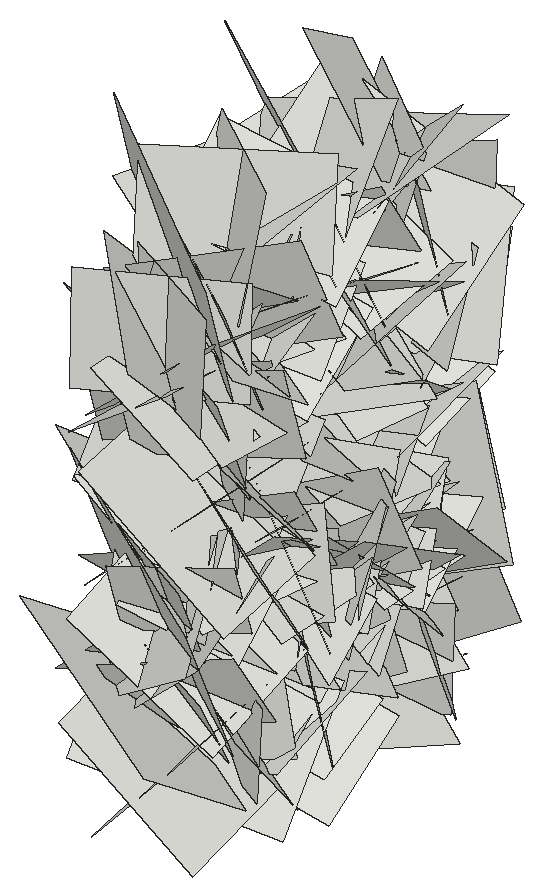
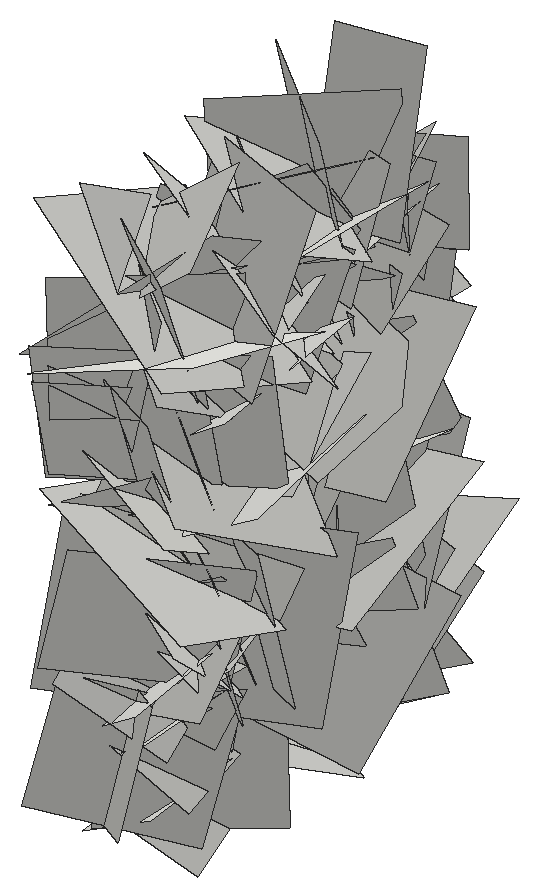
# SketchUp Ruby script. Lengths in inches.
U = 1.inch
M = Sketchup.active_model
def pt(a) = Geom::Point3d.new(a.map { |v| v * U })
def face(e, loops, mat)
  f = e.add_face(loops[0].map { |a| pt(a) })
  loops[1..].each { |l| e.add_face(l.map { |a| pt(a) }).erase! }
  f.material = f.back_material = mat if mat
  f
end
# faces: each face lists its corners as indices into pts; further lists are holes
def faces(e, pts, list, mat = nil) = list.each { |f| face(e, (f[0].is_a?(Array) ? f : [f]).map { |l| l.map { |i| pts[i] } }, mat) }
# xy, xz, yz: faces in a plane at the given z, y or x. An outline is a flat list of corners, or four numbers for a rectangle; further outlines are holes
def ring(l) = l.size == 4 ? [[l[0], l[1]], [l[2], l[1]], [l[2], l[3]], [l[0], l[3]]] : l.each_slice(2).to_a
def flat(e, list, mat, &to3) = list.each { |f| face(e, (f[0].is_a?(Array) ? f : [f]).map { |l| ring(l).map { |u, v| to3.(u, v) } }, mat) }
def xy(e, z, list, mat = nil) = flat(e, list, mat) { |x, y| [x, y, z] }
def xz(e, y, list, mat = nil) = flat(e, list, mat) { |x, z| [x, y, z] }
def yz(e, x, list, mat = nil) = flat(e, list, mat) { |y, z| [x, y, z] }
def lines(e, pts, list) = list.each { |a, b| e.add_line(pt(pts[a]), pt(pts[b])) }
# prism: a flat outline (further loops are holes) pulled along v
def prism(e, loops, v, mat = nil)
  f = face(e, loops, mat); d = Geom::Vector3d.new(v.map { |x| x * U })
  f.pushpull(f.normal.samedirection?(d) ? d.length : -d.length)
end
def box(e, o, s, mat = nil) = prism(e, [[o, [o[0] + s[0], o[1], o[2]], [o[0] + s[0], o[1] + s[1], o[2]], [o[0], o[1] + s[1], o[2]]]], [0, 0, s[2]], mat)
def at(x, y, z, deg = 0) = Geom::Transformation.translation(pt([x, y, z])) * Geom::Transformation.rotation(ORIGIN, Z_AXIS, deg.degrees)
def axes(o, x, y, z) = Geom::Transformation.new([*x, 0, *y, 0, *z, 0, *pt(o).to_a, 1])
def part(name) = M.definitions.add(name)
# library, detail: a bought-in or finely detailed component or shape, given as its bounding box
def library(name, o, s) = part(name).tap { |d| box(d.entities, o, s) }
def detail(e, o, s) = box(e.add_group.entities, o, s)
def put(e, d, t, mat = nil) = e.add_instance(d, t).tap { |i| i.material = mat if mat }
def group(e, t, mat = nil) = e.add_group.tap { |g| g.transformation = t; g.material = mat if mat }.entities
root = M.entities
c1 = part("Component\#6")
p = [[0.01,0,0],[0,3.24,4.54],[4.32,3.24,4.54],[4.33,0,0]]
faces(c1.entities,p,[[0,1,2,3]])
put(root,c1,axes([18.5,153.14,23.91],[-0.18,-1.08552,0.79109],[-0.08355,0.80406,1.08641],[-1.42134,0.0902,-0.16405]))
put(root,c1,axes([18.5,153.125,28.17],[0.03085,-0.9293,0.97672],[-0.26234,0.95667,0.91759],[-1.40479,-0.19906,-0.14991]))
put(root,c1,axes([18.5,153.73,28.3],[0.01858,0.99462,-0.84655],[-0.29457,-0.8244,-0.97435],[-1.35277,0.19318,0.20054]))
put(root,c1,axes([18.5,161.74,34.71],[-0.1652,-1.10091,-0.16395],[-0.26327,-0.12698,1.08875],[-1.15009,0.1872,-0.22568]))
put(root,c1,axes([18.5,157.5625,26.25],[-0.15158,-0.38022,-1.22414],[0.0526,-1.23246,0.37701],[-1.35773,-0.0053,0.15127]))
put(root,c1,axes([18.5,156.14,33.68],[-0.06217,-0.55405,1.15944],[-0.03014,1.16092,0.55332],[-1.36179,-0.0004,-0.06518]))
put(root,c1,axes([18.5,153.92,36.42],[-0.14295,0.82362,0.79821],[-0.11339,0.79118,-0.83443],[-1.21047,-0.17138,-0.0161]))
put(root,c1,axes([18.5,149.67,23.37],[0.09539,-0.59855,1.14231],[-0.08783,1.14003,0.60389],[-1.36418,-0.11525,0.041]))
put(root,c1,axes([18.5,150.2,21.48],[-0.03659,-0.96074,0.6365],[-0.08804,0.6372,0.9573],[-1.21843,-0.01719,-0.08829]))
put(root,c1,axes([18.5,152.25,36.24],[0.0137,1.21221,-0.26433],[-0.01965,-0.26413,-1.21218],[-1.31499,0.01657,0.01536]))
put(root,c1,axes([18.5,158.37,30.5],[-0.12568,-1.12455,0.31778],[0.06348,0.31314,1.13049],[-1.23707,0.13032,0.02572]))
put(root,c1,axes([18.5,156.79,29.67],[-0.01777,-0.29003,-1.18393],[0.05362,-1.18318,0.28913],[-1.29096,-0.04516,0.0283]))
put(root,c1,axes([18.5,155.57,33.875],[-0.13701,-1.11756,0.11199],[0.07264,0.10468,1.12363],[-1.18833,0.13525,0.05577]))
put(root,c1,axes([18.5,151.45,29.33],[-0.11063,1.17252,-0.59491],[0.28501,-0.56514,-1.16101],[-1.36425,-0.21315,-0.19431]))
put(root,c1,axes([18.5,153.58,31.99],[-0.17505,-0.32324,-0.90395],[-0.10086,-0.9072,0.34179],[-1.0126,0.14624,0.12223]))
put(root,c1,axes([18.5,157.84,26.69],[-0.16666,-0.37984,-0.88441],[-0.10341,-0.88523,0.39754],[-1.01503,0.15255,0.10471]))
put(root,c1,axes([18.5,160.05,30.35],[0.12426,0.20575,-1.35522],[0.11745,-1.35714,-0.19646],[-1.44825,-0.0924,-0.13221]))
put(root,c1,axes([18.5,158.93,27.77],[0.0679,-1.16178,0.21088],[-0.08573,0.20637,1.16154],[-1.24867,-0.07734,-0.06828]))
put(root,c1,axes([18.5,153.43,27.14],[-0.15407,-0.97446,-0.01303],[-0.08051,-0.00181,0.98239],[-1.02988,0.14592,-0.07485]))
put(root,c1,axes([18.5,147.58,26.68],[-0.22766,0.71104,0.67114],[0.02672,0.69094,-0.72395],[-1.03608,-0.13842,-0.16614]))
put(root,c1,axes([18.5,161.68,35.57],[0.09547,-0.29138,-1.10436],[-0.14499,-1.10257,0.27976],[-1.20197,0.10985,-0.12146]))
put(root,c1,axes([18.5,156.69,29.48],[0.02364,1.01192,0.31394],[-0.16386,0.31376,-1.00035],[-1.11105,-0.02474,0.15421]))
put(root,c1,axes([18.5,156.02,28.65],[0.0619,-0.85924,0.62732],[-0.17366,0.61351,0.85557],[-1.11425,-0.14335,-0.09849]))
put(root,c1,axes([14.53,160.09,33.87],[-0.13785,-0.16653,-0.67513],[-0.04892,-0.68326,0.17743],[0.73546,-0.07666,-0.11474]))
put(root,c1,axes([18.5,156.45,32.24],[-0.14884,0.843,-0.57449],[0.06248,-0.57223,-0.85409],[-1.07954,-0.14935,0.02978]))
put(root,c1,axes([14.53,157.4,31.875],[-0.05779,-0.51798,-0.36432],[-0.0587,-0.36037,0.52065],[0.6687,-0.0764,0.01422]))
put(root,c1,axes([14.53,149.08,38.35],[0.0057,0.54335,-0.52891],[-0.23788,-0.50408,-0.52014],[0.76776,-0.16022,-0.15723]))
put(root,c1,axes([18.5,152.14,28.92],[-0.00837,0.82237,-0.50147],[-0.16225,-0.49618,-0.8113],[-1.00803,0.07304,0.13474]))
put(root,c1,axes([18.5,154.59,24.16],[0.1724,0.15274,1.09758],[-0.17194,1.10067,-0.12914],[-1.16199,-0.14021,0.18195]))
put(root,c1,axes([14.53,157.59,40.82],[-0.16311,0.68993,-0.43022],[-0.09586,-0.44966,-0.68876],[0.85651,0.08106,-0.15901]))
put(root,c1,axes([18.5,154.4,23.625],[0.0407,-0.65785,-0.83395],[-0.03781,-0.83482,0.65689],[-1.12528,0.00426,-0.05223]))
put(root,c1,axes([14.53,158.03,24.73],[-0.19324,-0.05037,0.89121],[-0.15909,0.89838,0.02008],[0.93272,0.1428,0.18806]))
put(root,c1,axes([18.5,151.25,34.8],[-0.16779,0.3958,-0.75565],[-0.05631,-0.77163,-0.39305],[-0.90246,-0.02545,0.16502]))
put(root,c1,axes([18.5,159.15,23.91],[-0.14407,0.13595,-0.90237],[0.02833,-0.91134,-0.14133],[-0.9669,-0.04696,0.13032]))
put(root,c1,axes([14.53,161,38.46],[-0.19651,-0.13504,-0.81499],[-0.03185,-0.8336,0.14496],[0.87508,-0.06067,-0.17773]))
put(root,c1,axes([18.5,152.42,20.54],[0.05004,-0.6691,0.77955],[-0.05919,0.77755,0.67076],[-1.08735,-0.07312,-0.00064]))
put(root,c1,axes([18.5,154.96,37.56],[0.27688,1.1515,0.31839],[-0.11464,0.34737,-1.16756],[-1.26119,0.22122,0.17603]))
put(root,c1,axes([14.53,156.65,23.33],[0.01341,0.01203,0.69899],[-0.10657,0.69187,-0.01009],[0.73333,0.10033,-0.01425]))
put(root,c1,axes([18.5,158.66,27.8],[-0.19419,0.10037,-0.91545],[0.10975,-0.92523,-0.12216],[-0.97001,-0.12478,0.16945]))
put(root,c1,axes([14.53,158.73,27.09],[-0.13155,-0.14233,-0.74779],[-0.00006,-0.75766,0.14422],[0.80689,-0.02326,-0.12191]))
put(root,c1,axes([14.53,152.7,33.94],[-0.15183,0.13661,-0.74127],[0.04087,-0.75222,-0.14607],[0.79793,0.06452,-0.13357]))
put(root,c1,axes([18.5,149.65,34.23],[0.2234,-0.54463,1.08834],[0.02633,1.10624,0.54877],[-1.28976,-0.07175,0.19972]))
put(root,c1,axes([18.5,152.65,32.7],[0.31384,1.21799,0.62272],[0.13011,0.61092,-1.25326],[-1.44417,0.31973,0.02242]))
put(root,c1,axes([14.53,153.52,29.46],[-0.08102,0.00764,-0.81457],[-0.10707,-0.81193,0.00187],[0.85682,-0.10074,-0.07679]))
put(root,c1,axes([14.53,158.01,30.39],[0.08038,-0.60995,0.00551],[-0.02253,0.00291,0.6143],[0.64618,0.07598,0.02073]))
put(root,c1,axes([14.53,151.89,27.92],[0.07457,-0.37507,-0.49968],[-0.035,-0.50437,0.37394],[0.66135,0.0156,0.07613]))
put(root,c1,axes([18.5,158.65,23.12],[0.03,-0.65446,0.65644],[-0.11713,0.64968,0.65248],[-0.97555,-0.09812,-0.05816]))
put(root,c1,axes([14.53,150.81,32.67],[-0.03105,-0.70657,0.01303],[0.00041,0.01303,0.70717],[0.74909,-0.02929,0.00015]))
put(root,c1,axes([18.5,155.99,38.05],[-0.0315,0.52335,-0.79271],[0.01447,-0.79278,-0.52391],[-1.00678,-0.02777,0.01727]))
put(root,c1,axes([14.53,155.3,36.05],[-0.02231,-0.46484,-0.62566],[-0.10069,-0.6197,0.4636],[0.82005,-0.08874,0.0399]))
put(root,c1,axes([18.5,160.9375,37.33],[-0.13153,0.12633,-0.90974],[0.10231,-0.91113,-0.13969],[-0.96819,-0.11344,0.10882]))
put(root,c1,axes([18.5,153.79,24.7],[0.00565,-0.43188,0.90191],[0.04751,0.90112,0.43124],[-1.05892,0.03812,0.02416]))
put(root,c1,axes([18.5,152.27,30.34],[-0.04267,0.47891,-0.74389],[-0.05776,-0.74459,-0.47642],[-0.93603,0.02411,0.06331]))
put(root,c1,axes([18.5,150.92,33.45],[0.01124,-0.40239,0.85237],[-0.02564,0.85203,0.40253],[-0.99881,-0.0264,-0.00074]))
put(root,c1,axes([14.53,153.82,25.23],[0.04726,-0.11023,0.59197],[0.093,0.58845,0.10297],[0.63147,-0.07841,-0.05947]))
put(root,c1,axes([14.53,149.71,29.1],[0.04042,0.22115,-0.567],[0.10046,-0.56334,-0.21335],[0.63725,0.07479,0.0696]))
put(root,c1,axes([18.5,154.45,36.57],[-0.07713,0.81709,0.22722],[-0.03645,0.22503,-0.82021],[-0.89825,-0.07929,0.01378]))
put(root,c1,axes([14.53,158.75,26.14],[0.12859,0.59437,-0.23179],[-0.06253,-0.22448,-0.60651],[0.67335,-0.13435,-0.01206]))
put(root,c1,axes([18.5,156.72,22.08],[0.00521,-0.94479,0.50901],[0.17637,0.50353,0.93301],[-1.12382,0.07464,0.14878]))
put(root,c1,axes([14.53,156.34,37.48],[-0.20366,-0.78098,-0.33642],[0.07649,-0.35863,0.79133],[0.89812,-0.14656,-0.14368]))
put(root,c1,axes([18.5,150.56,37.37],[-0.01495,0.72639,-0.4873],[-0.06872,-0.48689,-0.7239],[-0.92463,0.02444,0.06168]))
put(root,c1,axes([14.53,156.49,28.09],[0.01227,0.36562,0.53928],[0.0952,0.53332,-0.36351],[0.68404,-0.08079,0.04092]))
put(root,c1,axes([18.5,150.4,30.92],[-0.04252,-0.27759,0.76161],[-0.13298,0.75548,0.26875],[-0.84891,-0.10444,-0.08025]))
put(root,c1,axes([18.5,152.31,24.83],[-0.14132,0.38772,0.61473],[-0.11706,0.60692,-0.40674],[-0.76145,-0.16526,-0.05156]))
put(root,c1,axes([14.53,150.69,21.46],[-0.08617,-0.06424,0.73191],[0.1147,0.7273,0.07585],[0.77031,-0.11548,0.07058]))
put(root,c1,axes([14.53,149.63,26.39],[-0.05575,0.3601,-0.58557],[0.15834,-0.56726,-0.36226],[0.71127,0.15451,0.03475]))
put(root,c1,axes([14.53,153.92,21.15],[-0.0271,-0.2919,0.8704],[-0.20523,0.85287,0.28034],[0.95124,0.17569,0.08528]))
put(root,c1,axes([14.53,159.1875,20.3125],[-0.01409,-0.35632,0.80543],[-0.16766,0.79339,0.34838],[0.91839,0.13938,0.07596]))
put(root,c1,axes([18.5,157.73,31.39],[0.13129,-0.92283,0.37392],[-0.04334,0.37177,0.93107],[-1.05456,-0.13017,0.00829]))
put(root,c1,axes([14.53,147.16,24.1],[-0.03025,0.92414,0.23442],[-0.23339,0.2218,-0.90118],[0.98329,0.08108,-0.20669]))
put(root,c1,axes([14.53,159.76,21.63],[0.09665,-0.666,0.12875],[-0.03078,0.12595,0.67212],[0.71837,0.095,0.01147]))
put(root,c1,axes([18.5,154.61,36.92],[0.07328,1.03426,0.55463],[0.26621,0.52968,-1.01904],[-1.21518,0.17841,-0.1898]))
put(root,c1,axes([14.53,160.84,30.26],[0.09118,-0.56201,-0.30691],[0.0596,-0.30185,0.56849],[0.67615,0.1024,-0.00872]))
put(root,c1,axes([14.53,156.05,22.34],[0.04217,-0.56806,-0.37659],[0.07293,-0.37196,0.56834],[0.71876,0.07107,-0.03557]))
put(root,c1,axes([18.5,158.82,28.52],[0.0834,-0.34729,-0.88838],[-0.00654,-0.89156,0.34799],[-1.01106,-0.02288,-0.07553]))
put(root,c1,axes([18.5,151.53,22],[0.08087,0.78957,0.40941],[-0.10212,0.41583,-0.78401],[-0.93722,0.02282,0.12075]))
put(root,c1,axes([18.5,152.86,25.21],[-0.07237,-0.84668,-0.40971],[0.16913,-0.41526,0.83156],[-0.98259,-0.00911,0.17331]))
put(root,c1,axes([18.5,150.44,37.52],[0.01758,-0.03984,-0.83316],[-0.08726,-0.82933,0.03802],[-0.87984,0.08145,-0.02042]))
put(root,c1,axes([18.5,161.57,34.4],[0.05292,-0.24359,-0.78611],[-0.1523,-0.77804,0.23197],[-0.85897,0.12294,-0.08956]))
put(root,c1,axes([14.53,154.14,39.875],[-0.07687,-0.17009,-0.90128],[-0.07958,-0.89996,0.17589],[0.96896,-0.0874,-0.05706]))
put(root,c1,axes([14.53,159.35,19.53],[0.12506,-0.65018,0.20227],[-0.00025,0.20525,0.65988],[0.72178,0.11273,-0.03482]))
put(root,c1,axes([18.5,155.63,34.51],[0.04715,-0.7148,-0.47013],[-0.06325,-0.47221,0.71232],[-0.90467,-0.00424,-0.0743]))
put(root,c1,axes([18.5,151.43,29.49],[0.01376,0.93036,0.01045],[0.09599,0.00914,-0.92605],[-0.98156,0.01394,-0.09041]))
put(root,c1,axes([18.5,156.02,27.27],[-0.01737,0.78195,0.05447],[-0.0729,0.05284,-0.77921],[-0.82768,-0.02106,0.06749]))
put(root,c1,axes([14.53,152.23,36.27],[0.17612,0.33723,0.58016],[-0.03508,0.60107,-0.33991],[0.71045,-0.05392,-0.16061]))
put(root,c1,axes([14.53,152.86,32.22],[-0.07765,-0.95123,0.12327],[-0.10469,0.13045,0.94796],[1.01133,-0.05954,0.1076]))
put(root,c1,axes([18.5,160.42,26.72],[0.04031,-0.6417,-0.5437],[-0.04231,-0.54502,0.64047],[-0.89052,-0.00315,-0.05504]))
put(root,c1,axes([14.53,153.18,27.99],[-0.08911,-1.01671,-0.11332],[-0.1646,-0.0997,1.00972],[1.07181,-0.09984,0.14565]))
put(root,c1,axes([18.5,153.18,27.99],[0.08911,-1.01671,-0.11332],[0.1646,-0.0997,1.00972],[-1.07181,-0.09984,0.14565]))
put(root,c1,axes([14.53,160.42,26.72],[-0.04031,-0.6417,-0.5437],[0.04231,-0.54502,0.64047],[0.89052,-0.00315,-0.05504]))
put(root,c1,axes([18.5,152.86,32.22],[0.07765,-0.95123,0.12327],[0.10469,0.13045,0.94796],[-1.01133,-0.05954,0.1076]))
put(root,c1,axes([18.5,152.23,36.27],[-0.17612,0.33723,0.58016],[0.03508,0.60107,-0.33991],[-0.71045,-0.05392,-0.16061]))
put(root,c1,axes([14.53,156.02,27.27],[0.01737,0.78195,0.05447],[0.0729,0.05284,-0.77921],[0.82768,-0.02106,0.06749]))
put(root,c1,axes([14.53,151.43,29.49],[-0.01376,0.93036,0.01045],[-0.09599,0.00914,-0.92605],[0.98156,0.01394,-0.09041]))
put(root,c1,axes([14.53,155.63,34.51],[-0.04715,-0.7148,-0.47013],[0.06325,-0.47221,0.71232],[0.90467,-0.00424,-0.0743]))
put(root,c1,axes([18.5,159.35,19.53],[-0.12506,-0.65018,0.20227],[0.00025,0.20525,0.65988],[-0.72178,0.11273,-0.03482]))
put(root,c1,axes([18.5,154.14,39.875],[0.07687,-0.17009,-0.90128],[0.07958,-0.89996,0.17589],[-0.96896,-0.0874,-0.05706]))
put(root,c1,axes([14.53,161.57,34.4],[-0.05292,-0.24359,-0.78611],[0.1523,-0.77804,0.23197],[0.85897,0.12294,-0.08956]))
put(root,c1,axes([14.53,150.44,37.52],[-0.01758,-0.03984,-0.83316],[0.08726,-0.82933,0.03802],[0.87984,0.08145,-0.02042]))
put(root,c1,axes([14.53,152.86,25.21],[0.07237,-0.84668,-0.40971],[-0.16913,-0.41526,0.83156],[0.98259,-0.00911,0.17331]))
put(root,c1,axes([14.53,151.53,22],[-0.08087,0.78957,0.40941],[0.10212,0.41583,-0.78401],[0.93722,0.02282,0.12075]))
put(root,c1,axes([14.53,158.82,28.52],[-0.0834,-0.34729,-0.88838],[0.00654,-0.89156,0.34799],[1.01106,-0.02288,-0.07553]))
put(root,c1,axes([18.5,156.05,22.34],[-0.04217,-0.56806,-0.37659],[-0.07293,-0.37196,0.56834],[-0.71876,0.07107,-0.03557]))
put(root,c1,axes([18.5,160.84,30.26],[-0.09118,-0.56201,-0.30691],[-0.0596,-0.30185,0.56849],[-0.67615,0.1024,-0.00872]))
put(root,c1,axes([14.53,154.61,36.92],[-0.07328,1.03426,0.55463],[-0.26621,0.52968,-1.01904],[1.21518,0.17841,-0.1898]))
put(root,c1,axes([18.5,159.76,21.63],[-0.09665,-0.666,0.12875],[0.03078,0.12595,0.67212],[-0.71837,0.095,0.01147]))
put(root,c1,axes([18.5,147.16,24.1],[0.03025,0.92414,0.23442],[0.23339,0.2218,-0.90118],[-0.98329,0.08108,-0.20669]))
put(root,c1,axes([14.53,157.73,31.39],[-0.13129,-0.92283,0.37392],[0.04334,0.37177,0.93107],[1.05456,-0.13017,0.00829]))
put(root,c1,axes([18.5,159.1875,20.3125],[0.01409,-0.35632,0.80543],[0.16766,0.79339,0.34838],[-0.91839,0.13938,0.07596]))
put(root,c1,axes([18.5,153.92,21.15],[0.0271,-0.2919,0.8704],[0.20523,0.85287,0.28034],[-0.95124,0.17569,0.08528]))
put(root,c1,axes([18.5,149.63,26.39],[0.05575,0.3601,-0.58557],[-0.15834,-0.56726,-0.36226],[-0.71127,0.15451,0.03475]))
put(root,c1,axes([18.5,150.69,21.46],[0.08617,-0.06424,0.73191],[-0.1147,0.7273,0.07585],[-0.77031,-0.11548,0.07058]))
put(root,c1,axes([14.53,152.31,24.83],[0.14132,0.38772,0.61473],[0.11706,0.60692,-0.40674],[0.76145,-0.16526,-0.05156]))
put(root,c1,axes([14.53,150.4,30.92],[0.04252,-0.27759,0.76161],[0.13298,0.75548,0.26875],[0.84891,-0.10444,-0.08025]))
put(root,c1,axes([18.5,156.49,28.09],[-0.01227,0.36562,0.53928],[-0.0952,0.53332,-0.36351],[-0.68404,-0.08079,0.04092]))
put(root,c1,axes([14.53,150.56,37.37],[0.01495,0.72639,-0.4873],[0.06872,-0.48689,-0.7239],[0.92463,0.02444,0.06168]))
put(root,c1,axes([18.5,156.34,37.48],[0.20366,-0.78098,-0.33642],[-0.07649,-0.35863,0.79133],[-0.89812,-0.14656,-0.14368]))
put(root,c1,axes([14.53,156.72,22.08],[-0.00521,-0.94479,0.50901],[-0.17637,0.50353,0.93301],[1.12382,0.07464,0.14878]))
put(root,c1,axes([18.5,158.75,26.14],[-0.12859,0.59437,-0.23179],[0.06253,-0.22448,-0.60651],[-0.67335,-0.13435,-0.01206]))
put(root,c1,axes([14.53,154.45,36.57],[0.07713,0.81709,0.22722],[0.03645,0.22503,-0.82021],[0.89825,-0.07929,0.01378]))
put(root,c1,axes([18.5,149.71,29.1],[-0.04042,0.22115,-0.567],[-0.10046,-0.56334,-0.21335],[-0.63725,0.07479,0.0696]))
put(root,c1,axes([18.5,153.82,25.23],[-0.04726,-0.11023,0.59197],[-0.093,0.58845,0.10297],[-0.63147,-0.07841,-0.05947]))
put(root,c1,axes([14.53,150.92,33.45],[-0.01124,-0.40239,0.85237],[0.02564,0.85203,0.40253],[0.99881,-0.0264,-0.00074]))
put(root,c1,axes([14.53,152.27,30.34],[0.04267,0.47891,-0.74389],[0.05776,-0.74459,-0.47642],[0.93603,0.02411,0.06331]))
put(root,c1,axes([14.53,153.79,24.7],[-0.00565,-0.43188,0.90191],[-0.04751,0.90112,0.43124],[1.05892,0.03812,0.02416]))
put(root,c1,axes([14.53,160.9375,37.33],[0.13153,0.12633,-0.90974],[-0.10231,-0.91113,-0.13969],[0.96819,-0.11344,0.10882]))
put(root,c1,axes([18.5,155.3,36.05],[0.02231,-0.46484,-0.62566],[0.10069,-0.6197,0.4636],[-0.82005,-0.08874,0.0399]))
put(root,c1,axes([14.53,155.99,38.05],[0.0315,0.52335,-0.79271],[-0.01447,-0.79278,-0.52391],[1.00678,-0.02777,0.01727]))
put(root,c1,axes([18.5,150.81,32.67],[0.03105,-0.70657,0.01303],[-0.00041,0.01303,0.70717],[-0.74909,-0.02929,0.00015]))
put(root,c1,axes([14.53,158.65,23.12],[-0.03,-0.65446,0.65644],[0.11713,0.64968,0.65248],[0.97555,-0.09812,-0.05816]))
put(root,c1,axes([18.5,151.89,27.92],[-0.07457,-0.37507,-0.49968],[0.035,-0.50437,0.37394],[-0.66135,0.0156,0.07613]))
put(root,c1,axes([18.5,158.01,30.39],[-0.08038,-0.60995,0.00551],[0.02253,0.00291,0.6143],[-0.64618,0.07598,0.02073]))
put(root,c1,axes([18.5,153.52,29.46],[0.08102,0.00764,-0.81457],[0.10707,-0.81193,0.00187],[-0.85682,-0.10074,-0.07679]))
